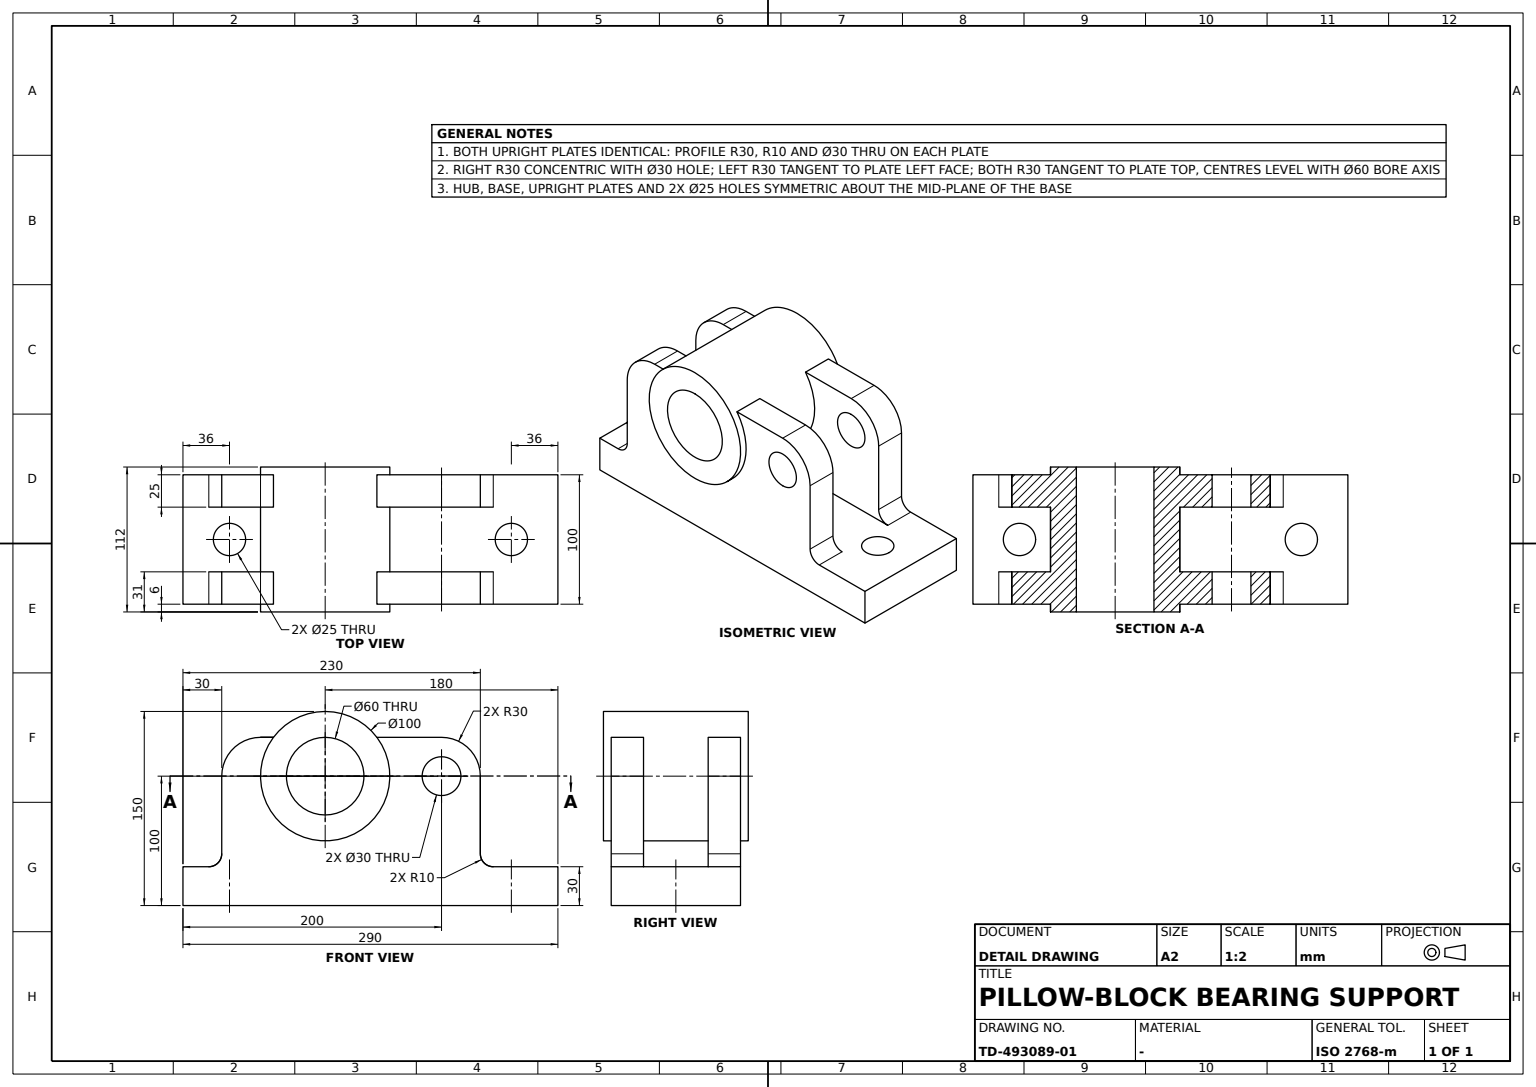
ISO-10303-21;
HEADER;
FILE_DESCRIPTION((''),'2;1');
FILE_NAME('','',(''),(''),'','','');
FILE_SCHEMA(('AUTOMOTIVE_DESIGN'));
ENDSEC;
DATA;
#1=APPLICATION_CONTEXT('');
#2=PRODUCT_CONTEXT('',#1,'mechanical');
#3=PRODUCT('','','',(#2));
#4=PRODUCT_DEFINITION_FORMATION('','',#3);
#5=PRODUCT_DEFINITION_CONTEXT('',#1,'design');
#6=PRODUCT_DEFINITION('','',#4,#5);
#7=PRODUCT_DEFINITION_SHAPE('','',#6);
#8=(LENGTH_UNIT()NAMED_UNIT(*)SI_UNIT(.MILLI.,.METRE.));
#9=(NAMED_UNIT(*)PLANE_ANGLE_UNIT()SI_UNIT($,.RADIAN.));
#10=(NAMED_UNIT(*)SI_UNIT($,.STERADIAN.)SOLID_ANGLE_UNIT());
#11=UNCERTAINTY_MEASURE_WITH_UNIT(LENGTH_MEASURE(0.005),#8,'distance_accuracy_value','');
#12=(GEOMETRIC_REPRESENTATION_CONTEXT(3)GLOBAL_UNCERTAINTY_ASSIGNED_CONTEXT((#11))GLOBAL_UNIT_ASSIGNED_CONTEXT((#8,#9,#10))REPRESENTATION_CONTEXT('',''));
#13=CARTESIAN_POINT('',(85.,-25.,40.000004));
#14=VERTEX_POINT('',#13);
#15=CARTESIAN_POINT('',(85.,-25.,100.));
#16=VERTEX_POINT('',#15);
#17=CARTESIAN_POINT('',(85.,-25.,30.));
#18=DIRECTION('',(0.,0.,1.));
#19=VECTOR('',#18,1000.);
#20=LINE('',#17,#19);
#21=EDGE_CURVE('',#14,#16,#20,.T.);
#22=ORIENTED_EDGE('',*,*,#21,.T.);
#23=CARTESIAN_POINT('',(85.,-50.,100.));
#24=VERTEX_POINT('',#23);
#25=CARTESIAN_POINT('',(85.,37.5,100.));
#26=DIRECTION('',(0.,-1.,0.));
#27=VECTOR('',#26,1000.);
#28=LINE('',#25,#27);
#29=EDGE_CURVE('',#16,#24,#28,.T.);
#30=ORIENTED_EDGE('',*,*,#29,.T.);
#31=CARTESIAN_POINT('',(85.,-50.,40.));
#32=VERTEX_POINT('',#31);
#33=CARTESIAN_POINT('',(85.,-50.,0.));
#34=LINE('',#33,#19);
#35=EDGE_CURVE('',#32,#24,#34,.T.);
#36=ORIENTED_EDGE('',*,*,#35,.F.);
#37=CARTESIAN_POINT('',(85.,0.,40.));
#38=LINE('',#37,#27);
#39=EDGE_CURVE('',#14,#32,#38,.T.);
#40=ORIENTED_EDGE('',*,*,#39,.F.);
#41=EDGE_LOOP('',(#22,#30,#36,#40));
#42=FACE_BOUND('',#41,.T.);
#43=CARTESIAN_POINT('',(85.,50.,30.));
#44=DIRECTION('',(1.,0.,0.));
#45=AXIS2_PLACEMENT_3D('',#43,#44,#18);
#46=PLANE('',#45);
#47=ADVANCED_FACE('',(#42),#46,.T.);
#48=CARTESIAN_POINT('',(55.,50.,85.));
#49=VERTEX_POINT('',#48);
#50=CARTESIAN_POINT('',(55.,50.,100.));
#51=DIRECTION('',(0.,0.,-1.));
#52=AXIS2_PLACEMENT_3D('',#50,#26,#51);
#53=CIRCLE('',#52,15.);
#54=EDGE_CURVE('',#49,#49,#53,.F.);
#55=ORIENTED_EDGE('',*,*,#54,.F.);
#56=EDGE_LOOP('',(#55));
#57=FACE_BOUND('',#56,.T.);
#58=CARTESIAN_POINT('',(145.,50.,0.));
#59=VERTEX_POINT('',#58);
#60=CARTESIAN_POINT('',(145.,50.,30.));
#61=VERTEX_POINT('',#60);
#62=LINE('',#58,#19);
#63=EDGE_CURVE('',#59,#61,#62,.T.);
#64=ORIENTED_EDGE('',*,*,#63,.F.);
#65=CARTESIAN_POINT('',(-145.,50.,0.));
#66=VERTEX_POINT('',#65);
#67=CARTESIAN_POINT('',(0.,50.,0.));
#68=VECTOR('',#44,1000.);
#69=LINE('',#67,#68);
#70=EDGE_CURVE('',#66,#59,#69,.T.);
#71=ORIENTED_EDGE('',*,*,#70,.F.);
#72=CARTESIAN_POINT('',(-145.,50.,30.));
#73=VERTEX_POINT('',#72);
#74=LINE('',#65,#19);
#75=EDGE_CURVE('',#66,#73,#74,.T.);
#76=ORIENTED_EDGE('',*,*,#75,.T.);
#77=CARTESIAN_POINT('',(-125.,50.,30.));
#78=VERTEX_POINT('',#77);
#79=CARTESIAN_POINT('',(0.,50.,30.));
#80=LINE('',#79,#68);
#81=EDGE_CURVE('',#73,#78,#80,.T.);
#82=ORIENTED_EDGE('',*,*,#81,.T.);
#83=CARTESIAN_POINT('',(-115.,50.,40.));
#84=VERTEX_POINT('',#83);
#85=CARTESIAN_POINT('',(-125.,50.,40.));
#86=AXIS2_PLACEMENT_3D('',#85,#26,#51);
#87=CIRCLE('',#86,10.);
#88=EDGE_CURVE('',#78,#84,#87,.T.);
#89=ORIENTED_EDGE('',*,*,#88,.T.);
#90=CARTESIAN_POINT('',(-115.,50.,100.));
#91=VERTEX_POINT('',#90);
#92=CARTESIAN_POINT('',(-115.,50.,0.));
#93=VECTOR('',#51,1000.);
#94=LINE('',#92,#93);
#95=EDGE_CURVE('',#91,#84,#94,.T.);
#96=ORIENTED_EDGE('',*,*,#95,.F.);
#97=CARTESIAN_POINT('',(-85.,50.,130.));
#98=VERTEX_POINT('',#97);
#99=CARTESIAN_POINT('',(-85.,50.,100.));
#100=AXIS2_PLACEMENT_3D('',#99,#26,#51);
#101=CIRCLE('',#100,30.);
#102=EDGE_CURVE('',#98,#91,#101,.T.);
#103=ORIENTED_EDGE('',*,*,#102,.F.);
#104=CARTESIAN_POINT('',(-75.,50.,130.));
#105=VERTEX_POINT('',#104);
#106=CARTESIAN_POINT('',(-145.,50.,130.));
#107=DIRECTION('',(-1.,0.,0.));
#108=VECTOR('',#107,1000.);
#109=LINE('',#106,#108);
#110=EDGE_CURVE('',#105,#98,#109,.T.);
#111=ORIENTED_EDGE('',*,*,#110,.F.);
#112=CARTESIAN_POINT('',(5.,50.,130.));
#113=VERTEX_POINT('',#112);
#114=CARTESIAN_POINT('',(-35.,50.,100.));
#115=AXIS2_PLACEMENT_3D('',#114,#26,#51);
#116=CIRCLE('',#115,50.);
#117=EDGE_CURVE('',#105,#113,#116,.T.);
#118=ORIENTED_EDGE('',*,*,#117,.T.);
#119=CARTESIAN_POINT('',(55.,50.,130.));
#120=VERTEX_POINT('',#119);
#121=EDGE_CURVE('',#120,#113,#109,.T.);
#122=ORIENTED_EDGE('',*,*,#121,.F.);
#123=CARTESIAN_POINT('',(85.,50.,100.));
#124=VERTEX_POINT('',#123);
#125=CIRCLE('',#52,30.);
#126=EDGE_CURVE('',#124,#120,#125,.T.);
#127=ORIENTED_EDGE('',*,*,#126,.F.);
#128=CARTESIAN_POINT('',(85.,50.,40.));
#129=VERTEX_POINT('',#128);
#130=CARTESIAN_POINT('',(85.,50.,0.));
#131=LINE('',#130,#19);
#132=EDGE_CURVE('',#129,#124,#131,.T.);
#133=ORIENTED_EDGE('',*,*,#132,.F.);
#134=CARTESIAN_POINT('',(95.,50.,30.));
#135=VERTEX_POINT('',#134);
#136=CARTESIAN_POINT('',(95.,50.,40.));
#137=AXIS2_PLACEMENT_3D('',#136,#26,#51);
#138=CIRCLE('',#137,10.);
#139=EDGE_CURVE('',#129,#135,#138,.T.);
#140=ORIENTED_EDGE('',*,*,#139,.T.);
#141=EDGE_CURVE('',#135,#61,#80,.T.);
#142=ORIENTED_EDGE('',*,*,#141,.T.);
#143=EDGE_LOOP('',(#64,#71,#76,#82,#89,#96,#103,#111,#118,#122,#127,#133,#140,#142));
#144=FACE_BOUND('',#143,.T.);
#145=AXIS2_PLACEMENT_3D('',#65,#26,#44);
#146=PLANE('',#145);
#147=ADVANCED_FACE('',(#57,#144),#146,.F.);
#148=CARTESIAN_POINT('',(55.,25.,130.));
#149=VERTEX_POINT('',#148);
#150=CARTESIAN_POINT('',(5.,25.,130.));
#151=VERTEX_POINT('',#150);
#152=CARTESIAN_POINT('',(85.,25.,130.));
#153=LINE('',#152,#108);
#154=EDGE_CURVE('',#149,#151,#153,.T.);
#155=ORIENTED_EDGE('',*,*,#154,.F.);
#156=CARTESIAN_POINT('',(55.,37.5,130.));
#157=LINE('',#156,#27);
#158=EDGE_CURVE('',#120,#149,#157,.T.);
#159=ORIENTED_EDGE('',*,*,#158,.F.);
#160=ORIENTED_EDGE('',*,*,#121,.T.);
#161=DIRECTION('',(0.,1.,0.));
#162=VECTOR('',#161,1000.);
#163=LINE('',#112,#162);
#164=EDGE_CURVE('',#113,#151,#163,.F.);
#165=ORIENTED_EDGE('',*,*,#164,.T.);
#166=EDGE_LOOP('',(#155,#159,#160,#165));
#167=FACE_BOUND('',#166,.T.);
#168=CARTESIAN_POINT('',(85.,50.,130.));
#169=AXIS2_PLACEMENT_3D('',#168,#18,#107);
#170=PLANE('',#169);
#171=ADVANCED_FACE('',(#167),#170,.T.);
#172=CARTESIAN_POINT('',(5.,-25.,130.));
#173=VERTEX_POINT('',#172);
#174=CARTESIAN_POINT('',(5.,-50.,130.));
#175=VERTEX_POINT('',#174);
#176=LINE('',#172,#162);
#177=EDGE_CURVE('',#173,#175,#176,.F.);
#178=ORIENTED_EDGE('',*,*,#177,.T.);
#179=CARTESIAN_POINT('',(55.,-50.,130.));
#180=VERTEX_POINT('',#179);
#181=CARTESIAN_POINT('',(-145.,-50.,130.));
#182=LINE('',#181,#108);
#183=EDGE_CURVE('',#180,#175,#182,.T.);
#184=ORIENTED_EDGE('',*,*,#183,.F.);
#185=CARTESIAN_POINT('',(55.,-25.,130.));
#186=VERTEX_POINT('',#185);
#187=EDGE_CURVE('',#186,#180,#157,.T.);
#188=ORIENTED_EDGE('',*,*,#187,.F.);
#189=CARTESIAN_POINT('',(85.,-25.,130.));
#190=LINE('',#189,#108);
#191=EDGE_CURVE('',#186,#173,#190,.T.);
#192=ORIENTED_EDGE('',*,*,#191,.T.);
#193=EDGE_LOOP('',(#178,#184,#188,#192));
#194=FACE_BOUND('',#193,.T.);
#195=ADVANCED_FACE('',(#194),#170,.T.);
#196=ORIENTED_EDGE('',*,*,#139,.F.);
#197=CARTESIAN_POINT('',(85.,25.,40.));
#198=VERTEX_POINT('',#197);
#199=EDGE_CURVE('',#129,#198,#38,.T.);
#200=ORIENTED_EDGE('',*,*,#199,.T.);
#201=CARTESIAN_POINT('',(95.,25.,30.));
#202=VERTEX_POINT('',#201);
#203=CARTESIAN_POINT('',(95.,25.,40.));
#204=AXIS2_PLACEMENT_3D('',#203,#161,#18);
#205=CIRCLE('',#204,10.);
#206=EDGE_CURVE('',#202,#198,#205,.T.);
#207=ORIENTED_EDGE('',*,*,#206,.F.);
#208=CARTESIAN_POINT('',(95.,0.,30.));
#209=LINE('',#208,#27);
#210=EDGE_CURVE('',#135,#202,#209,.T.);
#211=ORIENTED_EDGE('',*,*,#210,.F.);
#212=EDGE_LOOP('',(#196,#200,#207,#211));
#213=FACE_BOUND('',#212,.T.);
#214=CARTESIAN_POINT('',(95.,0.,40.));
#215=AXIS2_PLACEMENT_3D('',#214,#26,#107);
#216=CYLINDRICAL_SURFACE('',#215,10.);
#217=ADVANCED_FACE('',(#213),#216,.F.);
#218=CARTESIAN_POINT('',(55.,-50.,85.));
#219=VERTEX_POINT('',#218);
#220=CARTESIAN_POINT('',(55.,-50.,100.));
#221=AXIS2_PLACEMENT_3D('',#220,#26,#51);
#222=CIRCLE('',#221,15.);
#223=EDGE_CURVE('',#219,#219,#222,.T.);
#224=ORIENTED_EDGE('',*,*,#223,.F.);
#225=EDGE_LOOP('',(#224));
#226=FACE_BOUND('',#225,.T.);
#227=CARTESIAN_POINT('',(-75.,-50.,130.));
#228=VERTEX_POINT('',#227);
#229=CARTESIAN_POINT('',(-35.,-50.,100.));
#230=AXIS2_PLACEMENT_3D('',#229,#26,#51);
#231=CIRCLE('',#230,50.);
#232=EDGE_CURVE('',#228,#175,#231,.T.);
#233=ORIENTED_EDGE('',*,*,#232,.F.);
#234=CARTESIAN_POINT('',(-85.,-50.,130.));
#235=VERTEX_POINT('',#234);
#236=EDGE_CURVE('',#228,#235,#182,.T.);
#237=ORIENTED_EDGE('',*,*,#236,.T.);
#238=CARTESIAN_POINT('',(-115.,-50.,100.));
#239=VERTEX_POINT('',#238);
#240=CARTESIAN_POINT('',(-85.,-50.,100.));
#241=AXIS2_PLACEMENT_3D('',#240,#26,#51);
#242=CIRCLE('',#241,30.);
#243=EDGE_CURVE('',#235,#239,#242,.T.);
#244=ORIENTED_EDGE('',*,*,#243,.T.);
#245=CARTESIAN_POINT('',(-115.,-50.,40.000004));
#246=VERTEX_POINT('',#245);
#247=CARTESIAN_POINT('',(-115.,-50.,0.));
#248=LINE('',#247,#93);
#249=EDGE_CURVE('',#239,#246,#248,.T.);
#250=ORIENTED_EDGE('',*,*,#249,.T.);
#251=CARTESIAN_POINT('',(-125.,-50.,30.));
#252=VERTEX_POINT('',#251);
#253=CARTESIAN_POINT('',(-125.,-50.,40.));
#254=AXIS2_PLACEMENT_3D('',#253,#26,#51);
#255=CIRCLE('',#254,10.);
#256=EDGE_CURVE('',#252,#246,#255,.T.);
#257=ORIENTED_EDGE('',*,*,#256,.F.);
#258=CARTESIAN_POINT('',(-145.,-50.,30.));
#259=VERTEX_POINT('',#258);
#260=LINE('',#258,#108);
#261=EDGE_CURVE('',#252,#259,#260,.T.);
#262=ORIENTED_EDGE('',*,*,#261,.T.);
#263=CARTESIAN_POINT('',(-145.,-50.,0.));
#264=VERTEX_POINT('',#263);
#265=LINE('',#263,#19);
#266=EDGE_CURVE('',#264,#259,#265,.T.);
#267=ORIENTED_EDGE('',*,*,#266,.F.);
#268=CARTESIAN_POINT('',(145.,-50.,0.));
#269=VERTEX_POINT('',#268);
#270=LINE('',#263,#108);
#271=EDGE_CURVE('',#269,#264,#270,.T.);
#272=ORIENTED_EDGE('',*,*,#271,.F.);
#273=CARTESIAN_POINT('',(145.,-50.,30.));
#274=VERTEX_POINT('',#273);
#275=LINE('',#268,#19);
#276=EDGE_CURVE('',#269,#274,#275,.T.);
#277=ORIENTED_EDGE('',*,*,#276,.T.);
#278=CARTESIAN_POINT('',(95.000004,-50.,30.));
#279=VERTEX_POINT('',#278);
#280=EDGE_CURVE('',#274,#279,#260,.T.);
#281=ORIENTED_EDGE('',*,*,#280,.T.);
#282=CARTESIAN_POINT('',(95.,-50.,40.));
#283=AXIS2_PLACEMENT_3D('',#282,#26,#51);
#284=CIRCLE('',#283,10.);
#285=EDGE_CURVE('',#32,#279,#284,.T.);
#286=ORIENTED_EDGE('',*,*,#285,.F.);
#287=ORIENTED_EDGE('',*,*,#35,.T.);
#288=CIRCLE('',#221,30.);
#289=EDGE_CURVE('',#24,#180,#288,.T.);
#290=ORIENTED_EDGE('',*,*,#289,.T.);
#291=ORIENTED_EDGE('',*,*,#183,.T.);
#292=EDGE_LOOP('',(#233,#237,#244,#250,#257,#262,#267,#272,#277,#281,#286,#287,#290,#291));
#293=FACE_BOUND('',#292,.T.);
#294=AXIS2_PLACEMENT_3D('',#263,#26,#44);
#295=PLANE('',#294);
#296=ADVANCED_FACE('',(#226,#293),#295,.T.);
#297=CARTESIAN_POINT('',(-145.,0.,0.));
#298=LINE('',#297,#27);
#299=EDGE_CURVE('',#66,#264,#298,.T.);
#300=ORIENTED_EDGE('',*,*,#299,.T.);
#301=ORIENTED_EDGE('',*,*,#266,.T.);
#302=CARTESIAN_POINT('',(-145.,0.,30.));
#303=LINE('',#302,#27);
#304=EDGE_CURVE('',#73,#259,#303,.T.);
#305=ORIENTED_EDGE('',*,*,#304,.F.);
#306=ORIENTED_EDGE('',*,*,#75,.F.);
#307=EDGE_LOOP('',(#300,#301,#305,#306));
#308=FACE_BOUND('',#307,.T.);
#309=AXIS2_PLACEMENT_3D('',#65,#107,#26);
#310=PLANE('',#309);
#311=ADVANCED_FACE('',(#308),#310,.T.);
#312=CARTESIAN_POINT('',(-115.,-25.,40.));
#313=VERTEX_POINT('',#312);
#314=CARTESIAN_POINT('',(-115.,0.,40.));
#315=LINE('',#314,#27);
#316=EDGE_CURVE('',#313,#246,#315,.T.);
#317=ORIENTED_EDGE('',*,*,#316,.T.);
#318=ORIENTED_EDGE('',*,*,#249,.F.);
#319=CARTESIAN_POINT('',(-115.,-25.,100.));
#320=VERTEX_POINT('',#319);
#321=CARTESIAN_POINT('',(-115.,37.5,100.));
#322=LINE('',#321,#27);
#323=EDGE_CURVE('',#320,#239,#322,.T.);
#324=ORIENTED_EDGE('',*,*,#323,.F.);
#325=CARTESIAN_POINT('',(-115.,-25.,130.));
#326=LINE('',#325,#93);
#327=EDGE_CURVE('',#320,#313,#326,.T.);
#328=ORIENTED_EDGE('',*,*,#327,.T.);
#329=EDGE_LOOP('',(#317,#318,#324,#328));
#330=FACE_BOUND('',#329,.T.);
#331=CARTESIAN_POINT('',(-115.,50.,130.));
#332=AXIS2_PLACEMENT_3D('',#331,#107,#51);
#333=PLANE('',#332);
#334=ADVANCED_FACE('',(#330),#333,.T.);
#335=CARTESIAN_POINT('',(-75.,25.,130.));
#336=VERTEX_POINT('',#335);
#337=CARTESIAN_POINT('',(-85.,25.,130.));
#338=VERTEX_POINT('',#337);
#339=EDGE_CURVE('',#336,#338,#153,.T.);
#340=ORIENTED_EDGE('',*,*,#339,.T.);
#341=CARTESIAN_POINT('',(-115.,25.,100.));
#342=VERTEX_POINT('',#341);
#343=CARTESIAN_POINT('',(-85.,25.,100.));
#344=AXIS2_PLACEMENT_3D('',#343,#161,#18);
#345=CIRCLE('',#344,30.);
#346=EDGE_CURVE('',#342,#338,#345,.T.);
#347=ORIENTED_EDGE('',*,*,#346,.F.);
#348=CARTESIAN_POINT('',(-115.,25.,40.));
#349=VERTEX_POINT('',#348);
#350=CARTESIAN_POINT('',(-115.,25.,130.));
#351=LINE('',#350,#93);
#352=EDGE_CURVE('',#342,#349,#351,.T.);
#353=ORIENTED_EDGE('',*,*,#352,.T.);
#354=CARTESIAN_POINT('',(-125.,25.,30.));
#355=VERTEX_POINT('',#354);
#356=CARTESIAN_POINT('',(-125.,25.,40.));
#357=AXIS2_PLACEMENT_3D('',#356,#161,#18);
#358=CIRCLE('',#357,10.);
#359=EDGE_CURVE('',#349,#355,#358,.T.);
#360=ORIENTED_EDGE('',*,*,#359,.T.);
#361=CARTESIAN_POINT('',(0.,25.,30.));
#362=LINE('',#361,#68);
#363=EDGE_CURVE('',#355,#202,#362,.T.);
#364=ORIENTED_EDGE('',*,*,#363,.T.);
#365=ORIENTED_EDGE('',*,*,#206,.T.);
#366=CARTESIAN_POINT('',(85.,25.,100.));
#367=VERTEX_POINT('',#366);
#368=CARTESIAN_POINT('',(85.,25.,30.));
#369=LINE('',#368,#19);
#370=EDGE_CURVE('',#198,#367,#369,.T.);
#371=ORIENTED_EDGE('',*,*,#370,.T.);
#372=CARTESIAN_POINT('',(55.,25.,100.));
#373=AXIS2_PLACEMENT_3D('',#372,#161,#18);
#374=CIRCLE('',#373,30.);
#375=EDGE_CURVE('',#149,#367,#374,.T.);
#376=ORIENTED_EDGE('',*,*,#375,.F.);
#377=ORIENTED_EDGE('',*,*,#154,.T.);
#378=CARTESIAN_POINT('',(-35.,25.,100.));
#379=AXIS2_PLACEMENT_3D('',#378,#161,#18);
#380=CIRCLE('',#379,50.);
#381=EDGE_CURVE('',#151,#336,#380,.T.);
#382=ORIENTED_EDGE('',*,*,#381,.T.);
#383=EDGE_LOOP('',(#340,#347,#353,#360,#364,#365,#371,#376,#377,#382));
#384=FACE_BOUND('',#383,.T.);
#385=CARTESIAN_POINT('',(55.,25.,115.));
#386=VERTEX_POINT('',#385);
#387=CIRCLE('',#373,15.);
#388=EDGE_CURVE('',#386,#386,#387,.T.);
#389=ORIENTED_EDGE('',*,*,#388,.T.);
#390=EDGE_LOOP('',(#389));
#391=FACE_BOUND('',#390,.T.);
#392=CARTESIAN_POINT('',(0.,25.,0.));
#393=AXIS2_PLACEMENT_3D('',#392,#161,#107);
#394=PLANE('',#393);
#395=ADVANCED_FACE('',(#384,#391),#394,.F.);
#396=CARTESIAN_POINT('',(55.,-25.,115.));
#397=VERTEX_POINT('',#396);
#398=CARTESIAN_POINT('',(55.,-25.,100.));
#399=AXIS2_PLACEMENT_3D('',#398,#161,#18);
#400=CIRCLE('',#399,15.);
#401=EDGE_CURVE('',#397,#397,#400,.T.);
#402=ORIENTED_EDGE('',*,*,#401,.T.);
#403=EDGE_LOOP('',(#402));
#404=FACE_BOUND('',#403,.T.);
#405=ORIENTED_EDGE('',*,*,#223,.T.);
#406=EDGE_LOOP('',(#405));
#407=FACE_BOUND('',#406,.T.);
#408=CARTESIAN_POINT('',(55.,-3.66,100.));
#409=AXIS2_PLACEMENT_3D('',#408,#161,#107);
#410=CYLINDRICAL_SURFACE('',#409,15.);
#411=ADVANCED_FACE('',(#404,#407),#410,.F.);
#412=CARTESIAN_POINT('',(-75.,-25.,130.));
#413=VERTEX_POINT('',#412);
#414=LINE('',#412,#162);
#415=EDGE_CURVE('',#228,#413,#414,.T.);
#416=ORIENTED_EDGE('',*,*,#415,.T.);
#417=CARTESIAN_POINT('',(-85.,-25.,130.));
#418=VERTEX_POINT('',#417);
#419=EDGE_CURVE('',#413,#418,#190,.T.);
#420=ORIENTED_EDGE('',*,*,#419,.T.);
#421=CARTESIAN_POINT('',(-85.,37.5,130.));
#422=LINE('',#421,#27);
#423=EDGE_CURVE('',#418,#235,#422,.T.);
#424=ORIENTED_EDGE('',*,*,#423,.T.);
#425=ORIENTED_EDGE('',*,*,#236,.F.);
#426=EDGE_LOOP('',(#416,#420,#424,#425));
#427=FACE_BOUND('',#426,.T.);
#428=ADVANCED_FACE('',(#427),#170,.T.);
#429=ORIENTED_EDGE('',*,*,#256,.T.);
#430=ORIENTED_EDGE('',*,*,#316,.F.);
#431=CARTESIAN_POINT('',(-125.,-25.,30.));
#432=VERTEX_POINT('',#431);
#433=CARTESIAN_POINT('',(-125.,-25.,40.));
#434=AXIS2_PLACEMENT_3D('',#433,#161,#18);
#435=CIRCLE('',#434,10.);
#436=EDGE_CURVE('',#313,#432,#435,.T.);
#437=ORIENTED_EDGE('',*,*,#436,.T.);
#438=CARTESIAN_POINT('',(-125.,0.,30.));
#439=LINE('',#438,#27);
#440=EDGE_CURVE('',#432,#252,#439,.T.);
#441=ORIENTED_EDGE('',*,*,#440,.T.);
#442=EDGE_LOOP('',(#429,#430,#437,#441));
#443=FACE_BOUND('',#442,.T.);
#444=CARTESIAN_POINT('',(-125.,0.,40.));
#445=AXIS2_PLACEMENT_3D('',#444,#26,#51);
#446=CYLINDRICAL_SURFACE('',#445,10.);
#447=ADVANCED_FACE('',(#443),#446,.F.);
#448=CARTESIAN_POINT('',(-35.,56.,150.));
#449=VERTEX_POINT('',#448);
#450=CARTESIAN_POINT('',(-35.,56.,100.));
#451=AXIS2_PLACEMENT_3D('',#450,#161,#18);
#452=CIRCLE('',#451,50.);
#453=EDGE_CURVE('',#449,#449,#452,.T.);
#454=ORIENTED_EDGE('',*,*,#453,.F.);
#455=EDGE_LOOP('',(#454));
#456=FACE_BOUND('',#455,.T.);
#457=ORIENTED_EDGE('',*,*,#164,.F.);
#458=ORIENTED_EDGE('',*,*,#117,.F.);
#459=LINE('',#104,#162);
#460=EDGE_CURVE('',#336,#105,#459,.T.);
#461=ORIENTED_EDGE('',*,*,#460,.F.);
#462=ORIENTED_EDGE('',*,*,#381,.F.);
#463=EDGE_LOOP('',(#457,#458,#461,#462));
#464=FACE_BOUND('',#463,.T.);
#465=ORIENTED_EDGE('',*,*,#415,.F.);
#466=ORIENTED_EDGE('',*,*,#232,.T.);
#467=ORIENTED_EDGE('',*,*,#177,.F.);
#468=CARTESIAN_POINT('',(-35.,-25.,100.));
#469=AXIS2_PLACEMENT_3D('',#468,#161,#18);
#470=CIRCLE('',#469,50.);
#471=EDGE_CURVE('',#173,#413,#470,.T.);
#472=ORIENTED_EDGE('',*,*,#471,.T.);
#473=EDGE_LOOP('',(#465,#466,#467,#472));
#474=FACE_BOUND('',#473,.T.);
#475=CARTESIAN_POINT('',(-35.,-56.,150.));
#476=VERTEX_POINT('',#475);
#477=CARTESIAN_POINT('',(-35.,-56.,100.));
#478=AXIS2_PLACEMENT_3D('',#477,#161,#18);
#479=CIRCLE('',#478,50.);
#480=EDGE_CURVE('',#476,#476,#479,.T.);
#481=ORIENTED_EDGE('',*,*,#480,.T.);
#482=EDGE_LOOP('',(#481));
#483=FACE_BOUND('',#482,.T.);
#484=CARTESIAN_POINT('',(-35.,0.,100.));
#485=AXIS2_PLACEMENT_3D('',#484,#161,#107);
#486=CYLINDRICAL_SURFACE('',#485,50.);
#487=ADVANCED_FACE('',(#456,#464,#474,#483),#486,.T.);
#488=ORIENTED_EDGE('',*,*,#187,.T.);
#489=ORIENTED_EDGE('',*,*,#289,.F.);
#490=ORIENTED_EDGE('',*,*,#29,.F.);
#491=CIRCLE('',#399,30.);
#492=EDGE_CURVE('',#186,#16,#491,.T.);
#493=ORIENTED_EDGE('',*,*,#492,.F.);
#494=EDGE_LOOP('',(#488,#489,#490,#493));
#495=FACE_BOUND('',#494,.T.);
#496=CARTESIAN_POINT('',(55.,37.5,100.));
#497=AXIS2_PLACEMENT_3D('',#496,#26,#18);
#498=CYLINDRICAL_SURFACE('',#497,30.);
#499=ADVANCED_FACE('',(#495),#498,.T.);
#500=CARTESIAN_POINT('',(121.5,0.,0.));
#501=VERTEX_POINT('',#500);
#502=CARTESIAN_POINT('',(109.,0.,0.));
#503=AXIS2_PLACEMENT_3D('',#502,#18,#44);
#504=CIRCLE('',#503,12.5);
#505=EDGE_CURVE('',#501,#501,#504,.T.);
#506=ORIENTED_EDGE('',*,*,#505,.T.);
#507=EDGE_LOOP('',(#506));
#508=FACE_BOUND('',#507,.T.);
#509=ORIENTED_EDGE('',*,*,#271,.T.);
#510=ORIENTED_EDGE('',*,*,#299,.F.);
#511=ORIENTED_EDGE('',*,*,#70,.T.);
#512=CARTESIAN_POINT('',(145.,0.,0.));
#513=LINE('',#512,#162);
#514=EDGE_CURVE('',#269,#59,#513,.T.);
#515=ORIENTED_EDGE('',*,*,#514,.F.);
#516=EDGE_LOOP('',(#509,#510,#511,#515));
#517=FACE_BOUND('',#516,.T.);
#518=CARTESIAN_POINT('',(-96.5,0.,0.));
#519=VERTEX_POINT('',#518);
#520=CARTESIAN_POINT('',(-109.,0.,0.));
#521=AXIS2_PLACEMENT_3D('',#520,#18,#44);
#522=CIRCLE('',#521,12.5);
#523=EDGE_CURVE('',#519,#519,#522,.T.);
#524=ORIENTED_EDGE('',*,*,#523,.T.);
#525=EDGE_LOOP('',(#524));
#526=FACE_BOUND('',#525,.T.);
#527=CARTESIAN_POINT('',(0.,0.,0.));
#528=AXIS2_PLACEMENT_3D('',#527,#18,#44);
#529=PLANE('',#528);
#530=ADVANCED_FACE('',(#508,#517,#526),#529,.F.);
#531=ORIENTED_EDGE('',*,*,#401,.F.);
#532=EDGE_LOOP('',(#531));
#533=FACE_BOUND('',#532,.T.);
#534=CARTESIAN_POINT('',(95.,-25.,30.));
#535=VERTEX_POINT('',#534);
#536=CARTESIAN_POINT('',(0.,-25.,30.));
#537=LINE('',#536,#68);
#538=EDGE_CURVE('',#432,#535,#537,.T.);
#539=ORIENTED_EDGE('',*,*,#538,.F.);
#540=ORIENTED_EDGE('',*,*,#436,.F.);
#541=ORIENTED_EDGE('',*,*,#327,.F.);
#542=CARTESIAN_POINT('',(-85.,-25.,100.));
#543=AXIS2_PLACEMENT_3D('',#542,#161,#18);
#544=CIRCLE('',#543,30.);
#545=EDGE_CURVE('',#320,#418,#544,.T.);
#546=ORIENTED_EDGE('',*,*,#545,.T.);
#547=ORIENTED_EDGE('',*,*,#419,.F.);
#548=ORIENTED_EDGE('',*,*,#471,.F.);
#549=ORIENTED_EDGE('',*,*,#191,.F.);
#550=ORIENTED_EDGE('',*,*,#492,.T.);
#551=ORIENTED_EDGE('',*,*,#21,.F.);
#552=CARTESIAN_POINT('',(95.,-25.,40.));
#553=AXIS2_PLACEMENT_3D('',#552,#161,#18);
#554=CIRCLE('',#553,10.);
#555=EDGE_CURVE('',#535,#14,#554,.T.);
#556=ORIENTED_EDGE('',*,*,#555,.F.);
#557=EDGE_LOOP('',(#539,#540,#541,#546,#547,#548,#549,#550,#551,#556));
#558=FACE_BOUND('',#557,.T.);
#559=CARTESIAN_POINT('',(0.,-25.,0.));
#560=AXIS2_PLACEMENT_3D('',#559,#161,#107);
#561=PLANE('',#560);
#562=ADVANCED_FACE('',(#533,#558),#561,.T.);
#563=EDGE_CURVE('',#91,#342,#322,.T.);
#564=ORIENTED_EDGE('',*,*,#563,.T.);
#565=ORIENTED_EDGE('',*,*,#346,.T.);
#566=EDGE_CURVE('',#98,#338,#422,.T.);
#567=ORIENTED_EDGE('',*,*,#566,.F.);
#568=ORIENTED_EDGE('',*,*,#102,.T.);
#569=EDGE_LOOP('',(#564,#565,#567,#568));
#570=FACE_BOUND('',#569,.T.);
#571=CARTESIAN_POINT('',(-85.,37.5,100.));
#572=AXIS2_PLACEMENT_3D('',#571,#26,#107);
#573=CYLINDRICAL_SURFACE('',#572,30.);
#574=ADVANCED_FACE('',(#570),#573,.T.);
#575=ORIENTED_EDGE('',*,*,#453,.T.);
#576=EDGE_LOOP('',(#575));
#577=FACE_BOUND('',#576,.T.);
#578=CARTESIAN_POINT('',(-35.,56.,130.));
#579=VERTEX_POINT('',#578);
#580=CIRCLE('',#451,30.);
#581=EDGE_CURVE('',#579,#579,#580,.T.);
#582=ORIENTED_EDGE('',*,*,#581,.F.);
#583=EDGE_LOOP('',(#582));
#584=FACE_BOUND('',#583,.T.);
#585=CARTESIAN_POINT('',(0.,56.,0.));
#586=AXIS2_PLACEMENT_3D('',#585,#161,#107);
#587=PLANE('',#586);
#588=ADVANCED_FACE('',(#577,#584),#587,.T.);
#589=ORIENTED_EDGE('',*,*,#505,.F.);
#590=EDGE_LOOP('',(#589));
#591=FACE_BOUND('',#590,.T.);
#592=CARTESIAN_POINT('',(121.5,0.,30.));
#593=VERTEX_POINT('',#592);
#594=CARTESIAN_POINT('',(109.,0.,30.));
#595=AXIS2_PLACEMENT_3D('',#594,#18,#44);
#596=CIRCLE('',#595,12.5);
#597=EDGE_CURVE('',#593,#593,#596,.T.);
#598=ORIENTED_EDGE('',*,*,#597,.T.);
#599=EDGE_LOOP('',(#598));
#600=FACE_BOUND('',#599,.T.);
#601=CARTESIAN_POINT('',(109.,0.,14.34));
#602=AXIS2_PLACEMENT_3D('',#601,#18,#44);
#603=CYLINDRICAL_SURFACE('',#602,12.5);
#604=ADVANCED_FACE('',(#591,#600),#603,.F.);
#605=CARTESIAN_POINT('',(-35.,-56.,130.));
#606=VERTEX_POINT('',#605);
#607=CIRCLE('',#478,30.);
#608=EDGE_CURVE('',#606,#606,#607,.T.);
#609=ORIENTED_EDGE('',*,*,#608,.T.);
#610=EDGE_LOOP('',(#609));
#611=FACE_BOUND('',#610,.T.);
#612=ORIENTED_EDGE('',*,*,#480,.F.);
#613=EDGE_LOOP('',(#612));
#614=FACE_BOUND('',#613,.T.);
#615=CARTESIAN_POINT('',(0.,-56.,0.));
#616=AXIS2_PLACEMENT_3D('',#615,#161,#107);
#617=PLANE('',#616);
#618=ADVANCED_FACE('',(#611,#614),#617,.F.);
#619=EDGE_CURVE('',#78,#355,#439,.T.);
#620=ORIENTED_EDGE('',*,*,#619,.T.);
#621=ORIENTED_EDGE('',*,*,#359,.F.);
#622=EDGE_CURVE('',#84,#349,#315,.T.);
#623=ORIENTED_EDGE('',*,*,#622,.F.);
#624=ORIENTED_EDGE('',*,*,#88,.F.);
#625=EDGE_LOOP('',(#620,#621,#623,#624));
#626=FACE_BOUND('',#625,.T.);
#627=ADVANCED_FACE('',(#626),#446,.F.);
#628=ORIENTED_EDGE('',*,*,#566,.T.);
#629=ORIENTED_EDGE('',*,*,#339,.F.);
#630=ORIENTED_EDGE('',*,*,#460,.T.);
#631=ORIENTED_EDGE('',*,*,#110,.T.);
#632=EDGE_LOOP('',(#628,#629,#630,#631));
#633=FACE_BOUND('',#632,.T.);
#634=ADVANCED_FACE('',(#633),#170,.T.);
#635=EDGE_CURVE('',#535,#279,#209,.T.);
#636=ORIENTED_EDGE('',*,*,#635,.F.);
#637=ORIENTED_EDGE('',*,*,#555,.T.);
#638=ORIENTED_EDGE('',*,*,#39,.T.);
#639=ORIENTED_EDGE('',*,*,#285,.T.);
#640=EDGE_LOOP('',(#636,#637,#638,#639));
#641=FACE_BOUND('',#640,.T.);
#642=ADVANCED_FACE('',(#641),#216,.F.);
#643=ORIENTED_EDGE('',*,*,#563,.F.);
#644=ORIENTED_EDGE('',*,*,#95,.T.);
#645=ORIENTED_EDGE('',*,*,#622,.T.);
#646=ORIENTED_EDGE('',*,*,#352,.F.);
#647=EDGE_LOOP('',(#643,#644,#645,#646));
#648=FACE_BOUND('',#647,.T.);
#649=ADVANCED_FACE('',(#648),#333,.T.);
#650=ORIENTED_EDGE('',*,*,#581,.T.);
#651=EDGE_LOOP('',(#650));
#652=FACE_BOUND('',#651,.T.);
#653=ORIENTED_EDGE('',*,*,#608,.F.);
#654=EDGE_LOOP('',(#653));
#655=FACE_BOUND('',#654,.T.);
#656=CYLINDRICAL_SURFACE('',#485,30.);
#657=ADVANCED_FACE('',(#652,#655),#656,.F.);
#658=ORIENTED_EDGE('',*,*,#370,.F.);
#659=ORIENTED_EDGE('',*,*,#199,.F.);
#660=ORIENTED_EDGE('',*,*,#132,.T.);
#661=EDGE_CURVE('',#124,#367,#28,.T.);
#662=ORIENTED_EDGE('',*,*,#661,.T.);
#663=EDGE_LOOP('',(#658,#659,#660,#662));
#664=FACE_BOUND('',#663,.T.);
#665=ADVANCED_FACE('',(#664),#46,.T.);
#666=ORIENTED_EDGE('',*,*,#158,.T.);
#667=ORIENTED_EDGE('',*,*,#375,.T.);
#668=ORIENTED_EDGE('',*,*,#661,.F.);
#669=ORIENTED_EDGE('',*,*,#126,.T.);
#670=EDGE_LOOP('',(#666,#667,#668,#669));
#671=FACE_BOUND('',#670,.T.);
#672=ADVANCED_FACE('',(#671),#498,.T.);
#673=ORIENTED_EDGE('',*,*,#388,.F.);
#674=EDGE_LOOP('',(#673));
#675=FACE_BOUND('',#674,.T.);
#676=ORIENTED_EDGE('',*,*,#54,.T.);
#677=EDGE_LOOP('',(#676));
#678=FACE_BOUND('',#677,.T.);
#679=ADVANCED_FACE('',(#675,#678),#410,.F.);
#680=ORIENTED_EDGE('',*,*,#243,.F.);
#681=ORIENTED_EDGE('',*,*,#423,.F.);
#682=ORIENTED_EDGE('',*,*,#545,.F.);
#683=ORIENTED_EDGE('',*,*,#323,.T.);
#684=EDGE_LOOP('',(#680,#681,#682,#683));
#685=FACE_BOUND('',#684,.T.);
#686=ADVANCED_FACE('',(#685),#573,.T.);
#687=ORIENTED_EDGE('',*,*,#523,.F.);
#688=EDGE_LOOP('',(#687));
#689=FACE_BOUND('',#688,.T.);
#690=CARTESIAN_POINT('',(-96.5,0.,30.));
#691=VERTEX_POINT('',#690);
#692=CARTESIAN_POINT('',(-109.,0.,30.));
#693=AXIS2_PLACEMENT_3D('',#692,#18,#44);
#694=CIRCLE('',#693,12.5);
#695=EDGE_CURVE('',#691,#691,#694,.T.);
#696=ORIENTED_EDGE('',*,*,#695,.T.);
#697=EDGE_LOOP('',(#696));
#698=FACE_BOUND('',#697,.T.);
#699=CARTESIAN_POINT('',(-109.,0.,14.34));
#700=AXIS2_PLACEMENT_3D('',#699,#18,#44);
#701=CYLINDRICAL_SURFACE('',#700,12.5);
#702=ADVANCED_FACE('',(#689,#698),#701,.F.);
#703=ORIENTED_EDGE('',*,*,#261,.F.);
#704=ORIENTED_EDGE('',*,*,#440,.F.);
#705=ORIENTED_EDGE('',*,*,#538,.T.);
#706=ORIENTED_EDGE('',*,*,#635,.T.);
#707=ORIENTED_EDGE('',*,*,#280,.F.);
#708=CARTESIAN_POINT('',(145.,0.,30.));
#709=LINE('',#708,#162);
#710=EDGE_CURVE('',#274,#61,#709,.T.);
#711=ORIENTED_EDGE('',*,*,#710,.T.);
#712=ORIENTED_EDGE('',*,*,#141,.F.);
#713=ORIENTED_EDGE('',*,*,#210,.T.);
#714=ORIENTED_EDGE('',*,*,#363,.F.);
#715=ORIENTED_EDGE('',*,*,#619,.F.);
#716=ORIENTED_EDGE('',*,*,#81,.F.);
#717=ORIENTED_EDGE('',*,*,#304,.T.);
#718=EDGE_LOOP('',(#703,#704,#705,#706,#707,#711,#712,#713,#714,#715,#716,#717));
#719=FACE_BOUND('',#718,.T.);
#720=ORIENTED_EDGE('',*,*,#695,.F.);
#721=EDGE_LOOP('',(#720));
#722=FACE_BOUND('',#721,.T.);
#723=ORIENTED_EDGE('',*,*,#597,.F.);
#724=EDGE_LOOP('',(#723));
#725=FACE_BOUND('',#724,.T.);
#726=CARTESIAN_POINT('',(0.,0.,30.));
#727=AXIS2_PLACEMENT_3D('',#726,#18,#44);
#728=PLANE('',#727);
#729=ADVANCED_FACE('',(#719,#722,#725),#728,.T.);
#730=ORIENTED_EDGE('',*,*,#710,.F.);
#731=ORIENTED_EDGE('',*,*,#276,.F.);
#732=ORIENTED_EDGE('',*,*,#514,.T.);
#733=ORIENTED_EDGE('',*,*,#63,.T.);
#734=EDGE_LOOP('',(#730,#731,#732,#733));
#735=FACE_BOUND('',#734,.T.);
#736=AXIS2_PLACEMENT_3D('',#268,#44,#161);
#737=PLANE('',#736);
#738=ADVANCED_FACE('',(#735),#737,.T.);
#739=CLOSED_SHELL('',(#47,#147,#171,#195,#217,#296,#311,#334,#395,#411,#428,#447,#487,#499,#530,#562,#574,#588,#604,#618,#627,#634,#642,#649,#657,#665,#672,#679,#686,#702,#729,#738));
#740=MANIFOLD_SOLID_BREP('',#739);
#741=ADVANCED_BREP_SHAPE_REPRESENTATION('',(#740),#12);
#742=SHAPE_DEFINITION_REPRESENTATION(#7,#741);
ENDSEC;
END-ISO-10303-21;
